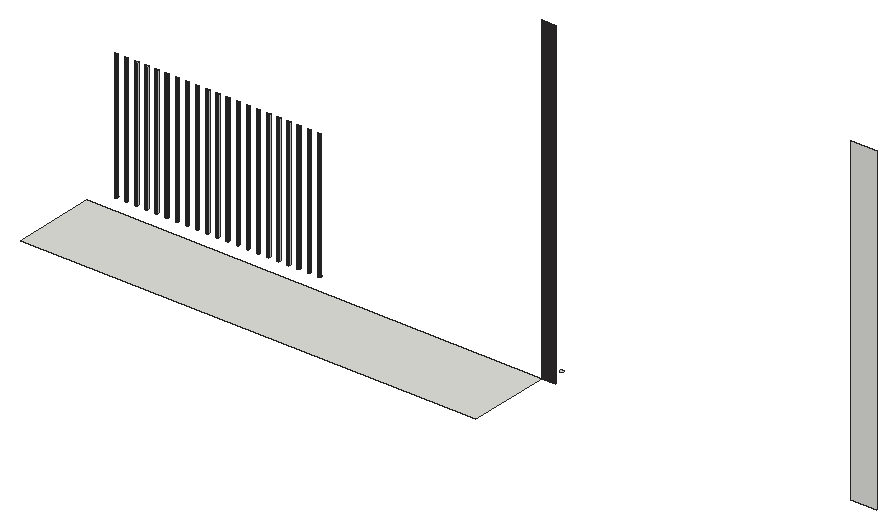
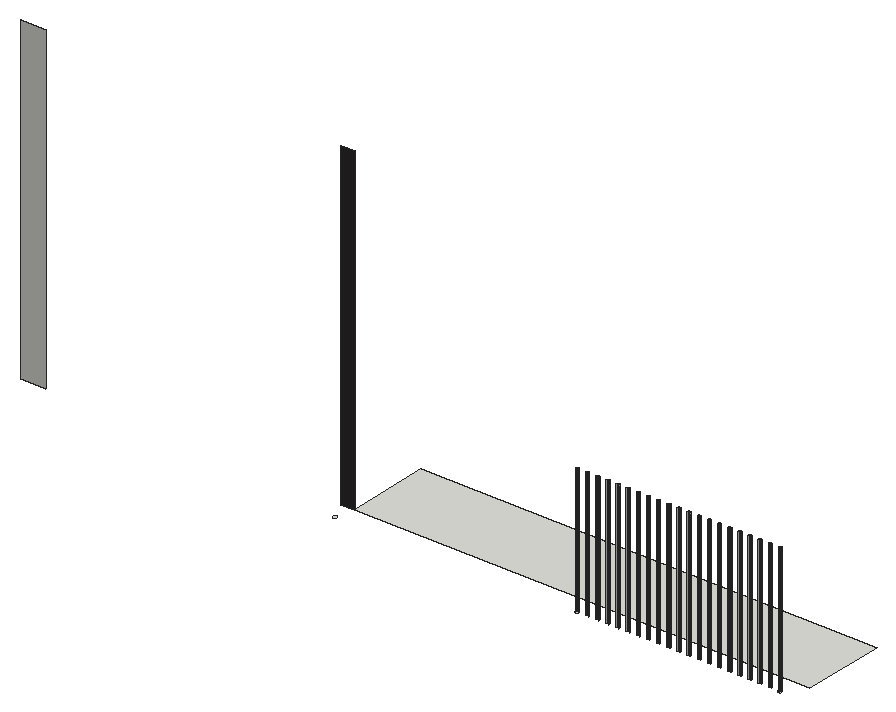
# SketchUp Ruby script. Lengths in inches.
U = 1.inch
M = Sketchup.active_model
def pt(a) = Geom::Point3d.new(a.map { |v| v * U })
def face(e, loops, mat)
  f = e.add_face(loops[0].map { |a| pt(a) })
  loops[1..].each { |l| e.add_face(l.map { |a| pt(a) }).erase! }
  f.material = f.back_material = mat if mat
  f
end
# faces: each face lists its corners as indices into pts; further lists are holes
def faces(e, pts, list, mat = nil) = list.each { |f| face(e, (f[0].is_a?(Array) ? f : [f]).map { |l| l.map { |i| pts[i] } }, mat) }
# xy, xz, yz: faces in a plane at the given z, y or x. An outline is a flat list of corners, or four numbers for a rectangle; further outlines are holes
def ring(l) = l.size == 4 ? [[l[0], l[1]], [l[2], l[1]], [l[2], l[3]], [l[0], l[3]]] : l.each_slice(2).to_a
def flat(e, list, mat, &to3) = list.each { |f| face(e, (f[0].is_a?(Array) ? f : [f]).map { |l| ring(l).map { |u, v| to3.(u, v) } }, mat) }
def xy(e, z, list, mat = nil) = flat(e, list, mat) { |x, y| [x, y, z] }
def xz(e, y, list, mat = nil) = flat(e, list, mat) { |x, z| [x, y, z] }
def yz(e, x, list, mat = nil) = flat(e, list, mat) { |y, z| [x, y, z] }
def lines(e, pts, list) = list.each { |a, b| e.add_line(pt(pts[a]), pt(pts[b])) }
# prism: a flat outline (further loops are holes) pulled along v
def prism(e, loops, v, mat = nil)
  f = face(e, loops, mat); d = Geom::Vector3d.new(v.map { |x| x * U })
  f.pushpull(f.normal.samedirection?(d) ? d.length : -d.length)
end
def box(e, o, s, mat = nil) = prism(e, [[o, [o[0] + s[0], o[1], o[2]], [o[0] + s[0], o[1] + s[1], o[2]], [o[0], o[1] + s[1], o[2]]]], [0, 0, s[2]], mat)
def at(x, y, z, deg = 0) = Geom::Transformation.translation(pt([x, y, z])) * Geom::Transformation.rotation(ORIGIN, Z_AXIS, deg.degrees)
def axes(o, x, y, z) = Geom::Transformation.new([*x, 0, *y, 0, *z, 0, *pt(o).to_a, 1])
def part(name) = M.definitions.add(name)
# library, detail: a bought-in or finely detailed component or shape, given as its bounding box
def library(name, o, s) = part(name).tap { |d| box(d.entities, o, s) }
def detail(e, o, s) = box(e.add_group.entities, o, s)
def put(e, d, t, mat = nil) = e.add_instance(d, t).tap { |i| i.material = mat if mat }
def group(e, t, mat = nil) = e.add_group.tap { |g| g.transformation = t; g.material = mat if mat }.entities
root = M.entities
M.materials.add("Generic\#4").color = [48, 45, 45]
xy(root,409.875,[[290.4375,81.125,528.75,124.5],[298.29,133.41,298.08,133.44,297.89,133.52,297.72,133.65,297.59,133.82,297.51,134.02,297.48,134.23,297.51,134.4375,297.59,134.63,297.72,134.8,297.89,134.93,298.08,135.01,298.29,135.04,298.5,135.01,298.7,134.93,298.87,134.8,299,134.63,299.08,134.4375,299.11,134.23,299.08,134.02,299,133.82,298.87,133.65,298.7,133.52,298.5,133.44],[404.54,133.41,404.33,133.44,404.14,133.52,403.97,133.65,403.84,133.82,403.76,134.02,403.73,134.23,403.76,134.4375,403.84,134.63,403.97,134.8,404.14,134.93,404.33,135.01,404.54,135.04,404.75,135.01,404.95,134.93,405.12,134.8,405.25,134.63,405.33,134.4375,405.36,134.23,405.33,134.02,405.25,133.82,405.12,133.65,404.95,133.52,404.75,133.44],[531.17,133.41,530.96,133.44,530.76,133.52,530.59,133.65,530.46,133.82,530.38,134.02,530.36,134.23,530.38,134.4375,530.46,134.63,530.59,134.8,530.76,134.93,530.96,135.01,531.17,135.04,531.38,135.01,531.57,134.93,531.74,134.8,531.87,134.63,531.95,134.4375,531.98,134.23,531.95,134.02,531.87,133.82,531.74,133.65,531.57,133.52,531.38,133.44]])
xz(root,124.5,[[690.4375,409.875,703.6875,577.875]])
xz(root,124.5,[[528.75,409.875,535.75,577.875]],"Generic\#4")
p = [[297.89,133.52,409.875],[298.08,133.44,409.875],[298.08,133.44,477.08],[297.89,133.52,477.08],[298.29,133.41,409.875],[298.29,133.41,477.08],
  [298.5,133.44,409.875],[298.5,133.44,477.08],[298.7,133.52,409.875],[298.7,133.52,477.08],[303.2,133.52,409.875],[303.4,133.44,409.875],
  [303.4,133.44,477.08],[303.2,133.52,477.08],[303.61,133.41,409.875],[303.61,133.41,477.08],[303.82,133.44,409.875],[303.82,133.44,477.08],
  [304.01,133.52,409.875],[304.01,133.52,477.08],[308.51,133.52,409.875],[308.71,133.44,409.875],[308.71,133.44,477.08],[308.51,133.52,477.08],
  [308.92,133.41,409.875],[308.92,133.41,477.08],[309.13,133.44,409.875],[309.13,133.44,477.08],[309.32,133.52,409.875],[309.32,133.52,477.08],
  [313.82,133.52,409.875],[314.02,133.44,409.875],[314.02,133.44,477.08],[313.82,133.52,477.08],[314.23,133.41,409.875],[314.23,133.41,477.08],
  [314.44,133.44,409.875],[314.44,133.44,477.08],[314.64,133.52,409.875],[314.64,133.52,477.08],[319.14,133.52,409.875],[319.33,133.44,409.875],
  [319.33,133.44,477.08],[319.14,133.52,477.08],[319.54,133.41,409.875],[319.54,133.41,477.08],[319.75,133.44,409.875],[319.75,133.44,477.08],
  [319.95,133.52,409.875],[319.95,133.52,477.08],[324.45,133.52,409.875],[324.65,133.44,409.875],[324.65,133.44,477.08],[324.45,133.52,477.08],
  [324.86,133.41,409.875],[324.86,133.41,477.08],[325.07,133.44,409.875],[325.07,133.44,477.08],[325.26,133.52,409.875],[325.26,133.52,477.08],
  [329.76,133.52,409.875],[329.96,133.44,409.875],[329.96,133.44,477.08],[329.76,133.52,477.08],[330.17,133.41,409.875],[330.17,133.41,477.08],
  [330.38,133.44,409.875],[330.38,133.44,477.08],[330.57,133.52,409.875],[330.57,133.52,477.08],[335.07,133.52,409.875],[335.27,133.44,409.875],
  [335.27,133.44,477.08],[335.07,133.52,477.08],[335.48,133.41,409.875],[335.48,133.41,477.08],[335.69,133.44,409.875],[335.69,133.44,477.08],
  [335.89,133.52,409.875],[335.89,133.52,477.08],[340.39,133.52,409.875],[340.58,133.44,409.875],[340.58,133.44,477.08],[340.39,133.52,477.08],
  [340.79,133.41,409.875],[340.79,133.41,477.08],[341,133.44,409.875],[341,133.44,477.08],[341.2,133.52,409.875],[341.2,133.52,477.08],
  [345.7,133.52,409.875],[345.9,133.44,409.875],[345.9,133.44,477.08],[345.7,133.52,477.08],[346.11,133.41,409.875],[346.11,133.41,477.08],
  [346.32,133.44,409.875],[346.32,133.44,477.08],[346.51,133.52,409.875],[346.51,133.52,477.08],[351.01,133.52,409.875],[351.21,133.44,409.875],
  [351.21,133.44,477.08],[351.01,133.52,477.08],[351.42,133.41,409.875],[351.42,133.41,477.08],[351.63,133.44,409.875],[351.63,133.44,477.08],
  [351.82,133.52,409.875],[351.82,133.52,477.08],[356.32,133.52,409.875],[356.52,133.44,409.875],[356.52,133.44,477.08],[356.32,133.52,477.08],
  [356.73,133.41,409.875],[356.73,133.41,477.08],[356.94,133.44,409.875],[356.94,133.44,477.08],[357.14,133.52,409.875],[357.14,133.52,477.08],
  [361.64,133.52,409.875],[361.83,133.44,409.875],[361.83,133.44,477.08],[361.64,133.52,477.08],[362.04,133.41,409.875],[362.04,133.41,477.08],
  [362.25,133.44,409.875],[362.25,133.44,477.08],[362.45,133.52,409.875],[362.45,133.52,477.08],[366.95,133.52,409.875],[367.15,133.44,409.875],
  [367.15,133.44,477.08],[366.95,133.52,477.08],[367.36,133.41,409.875],[367.36,133.41,477.08],[367.57,133.44,409.875],[367.57,133.44,477.08],
  [367.76,133.52,409.875],[367.76,133.52,477.08],[372.26,133.52,409.875],[372.46,133.44,409.875],[372.46,133.44,477.08],[372.26,133.52,477.08],
  [372.67,133.41,409.875],[372.67,133.41,477.08],[372.88,133.44,409.875],[372.88,133.44,477.08],[373.07,133.52,409.875],[373.07,133.52,477.08],
  [377.57,133.52,409.875],[377.77,133.44,409.875],[377.77,133.44,477.08],[377.57,133.52,477.08],[377.98,133.41,409.875],[377.98,133.41,477.08],
  [378.19,133.44,409.875],[378.19,133.44,477.08],[378.39,133.52,409.875],[378.39,133.52,477.08],[382.89,133.52,409.875],[383.08,133.44,409.875],
  [383.08,133.44,477.08],[382.89,133.52,477.08],[383.29,133.41,409.875],[383.29,133.41,477.08],[383.5,133.44,409.875],[383.5,133.44,477.08],
  [383.7,133.52,409.875],[383.7,133.52,477.08],[388.2,133.52,409.875],[388.4,133.44,409.875],[388.4,133.44,477.08],[388.2,133.52,477.08],
  [388.61,133.41,409.875],[388.61,133.41,477.08],[388.82,133.44,409.875],[388.82,133.44,477.08],[389.01,133.52,409.875],[389.01,133.52,477.08],
  [393.51,133.52,409.875],[393.71,133.44,409.875],[393.71,133.44,477.08],[393.51,133.52,477.08],[393.92,133.41,409.875],[393.92,133.41,477.08],
  [394.13,133.44,409.875],[394.13,133.44,477.08],[394.32,133.52,409.875],[394.32,133.52,477.08],[398.82,133.52,409.875],[399.02,133.44,409.875],
  [399.02,133.44,477.08],[398.82,133.52,477.08],[399.23,133.41,409.875],[399.23,133.41,477.08],[399.44,133.44,409.875],[399.44,133.44,477.08],
  [399.64,133.52,409.875],[399.64,133.52,477.08],[404.14,133.52,409.875],[404.33,133.44,409.875],[404.33,133.44,477.08],[404.14,133.52,477.08],
  [404.54,133.41,409.875],[404.54,133.41,477.08],[404.75,133.44,409.875],[404.75,133.44,477.08],[404.95,133.52,409.875],[404.95,133.52,477.08],
  [297.72,133.65,409.875],[297.72,133.65,477.08],[298.87,133.65,409.875],[298.87,133.65,477.08],[303.03,133.65,409.875],[303.03,133.65,477.08],
  [304.18,133.65,409.875],[304.18,133.65,477.08],[308.34,133.65,409.875],[308.34,133.65,477.08],[309.49,133.65,409.875],[309.49,133.65,477.08],
  [313.66,133.65,409.875],[313.66,133.65,477.08],[314.8,133.65,409.875],[314.8,133.65,477.08],[318.97,133.65,409.875],[318.97,133.65,477.08],
  [320.12,133.65,409.875],[320.12,133.65,477.08],[324.28,133.65,409.875],[324.28,133.65,477.08],[325.43,133.65,409.875],[325.43,133.65,477.08],
  [329.59,133.65,409.875],[329.59,133.65,477.08],[330.74,133.65,409.875],[330.74,133.65,477.08],[334.91,133.65,409.875],[334.91,133.65,477.08],
  [336.05,133.65,409.875],[336.05,133.65,477.08],[340.22,133.65,409.875],[340.22,133.65,477.08],[341.37,133.65,409.875],[341.37,133.65,477.08],
  [345.53,133.65,409.875],[345.53,133.65,477.08],[346.68,133.65,409.875],[346.68,133.65,477.08],[350.84,133.65,409.875],[350.84,133.65,477.08],
  [351.99,133.65,409.875],[351.99,133.65,477.08],[356.16,133.65,409.875],[356.16,133.65,477.08],[357.3,133.65,409.875],[357.3,133.65,477.08],
  [361.47,133.65,409.875],[361.47,133.65,477.08],[362.62,133.65,409.875],[362.62,133.65,477.08],[366.78,133.65,409.875],[366.78,133.65,477.08],
  [367.93,133.65,409.875],[367.93,133.65,477.08],[372.09,133.65,409.875],[372.09,133.65,477.08],[373.24,133.65,409.875],[373.24,133.65,477.08],
  [377.41,133.65,409.875],[377.41,133.65,477.08],[378.55,133.65,409.875],[378.55,133.65,477.08],[382.72,133.65,409.875],[382.72,133.65,477.08],
  [383.87,133.65,409.875],[383.87,133.65,477.08],[388.03,133.65,409.875],[388.03,133.65,477.08],[389.18,133.65,409.875],[389.18,133.65,477.08],
  [393.34,133.65,409.875],[393.34,133.65,477.08],[394.49,133.65,409.875],[394.49,133.65,477.08],[398.66,133.65,409.875],[398.66,133.65,477.08],
  [399.8,133.65,409.875],[399.8,133.65,477.08],[403.97,133.65,409.875],[403.97,133.65,477.08],[405.12,133.65,409.875],[405.12,133.65,477.08],
  [297.59,133.82,409.875],[297.59,133.82,477.08],[299,133.82,409.875],[299,133.82,477.08],[302.9,133.82,409.875],[302.9,133.82,477.08],
  [304.31,133.82,409.875],[304.31,133.82,477.08],[308.21,133.82,409.875],[308.21,133.82,477.08],[309.62,133.82,409.875],[309.62,133.82,477.08],
  [313.53,133.82,409.875],[313.53,133.82,477.08],[314.93,133.82,409.875],[314.93,133.82,477.08],[318.84,133.82,409.875],[318.84,133.82,477.08],
  [320.25,133.82,409.875],[320.25,133.82,477.08],[324.15,133.82,409.875],[324.15,133.82,477.08],[325.56,133.82,409.875],[325.56,133.82,477.08],
  [329.46,133.82,409.875],[329.46,133.82,477.08],[330.87,133.82,409.875],[330.87,133.82,477.08],[334.78,133.82,409.875],[334.78,133.82,477.08],
  [336.18,133.82,409.875],[336.18,133.82,477.08],[340.09,133.82,409.875],[340.09,133.82,477.08],[341.5,133.82,409.875],[341.5,133.82,477.08],
  [345.4,133.82,409.875],[345.4,133.82,477.08],[346.81,133.82,409.875],[346.81,133.82,477.08],[350.71,133.82,409.875],[350.71,133.82,477.08],
  [352.12,133.82,409.875],[352.12,133.82,477.08],[356.03,133.82,409.875],[356.03,133.82,477.08],[357.43,133.82,409.875],[357.43,133.82,477.08],
  [361.34,133.82,409.875],[361.34,133.82,477.08],[362.75,133.82,409.875],[362.75,133.82,477.08],[366.65,133.82,409.875],[366.65,133.82,477.08],
  [368.06,133.82,409.875],[368.06,133.82,477.08],[371.96,133.82,409.875],[371.96,133.82,477.08],[373.37,133.82,409.875],[373.37,133.82,477.08],
  [377.28,133.82,409.875],[377.28,133.82,477.08],[378.68,133.82,409.875],[378.68,133.82,477.08],[382.59,133.82,409.875],[382.59,133.82,477.08],
  [384,133.82,409.875],[384,133.82,477.08],[387.9,133.82,409.875],[387.9,133.82,477.08],[389.31,133.82,409.875],[389.31,133.82,477.08],
  [393.21,133.82,409.875],[393.21,133.82,477.08],[394.62,133.82,409.875],[394.62,133.82,477.08],[398.53,133.82,409.875],[398.53,133.82,477.08],
  [399.93,133.82,409.875],[399.93,133.82,477.08],[403.84,133.82,409.875],[403.84,133.82,477.08],[405.25,133.82,409.875],[405.25,133.82,477.08],
  [297.51,134.02,409.875],[297.51,134.02,477.08],[299.08,134.02,409.875],[299.08,134.02,477.08],[302.82,134.02,409.875],[302.82,134.02,477.08],
  [304.39,134.02,409.875],[304.39,134.02,477.08],[308.13,134.02,409.875],[308.13,134.02,477.08],[309.7,134.02,409.875],[309.7,134.02,477.08],
  [313.45,134.02,409.875],[313.45,134.02,477.08],[315.02,134.02,409.875],[315.02,134.02,477.08],[318.76,134.02,409.875],[318.76,134.02,477.08],
  [320.33,134.02,409.875],[320.33,134.02,477.08],[324.07,134.02,409.875],[324.07,134.02,477.08],[325.64,134.02,409.875],[325.64,134.02,477.08],
  [329.38,134.02,409.875],[329.38,134.02,477.08],[330.95,134.02,409.875],[330.95,134.02,477.08],[334.7,134.02,409.875],[334.7,134.02,477.08],
  [336.27,134.02,409.875],[336.27,134.02,477.08],[340.01,134.02,409.875],[340.01,134.02,477.08],[341.58,134.02,409.875],[341.58,134.02,477.08],
  [345.32,134.02,409.875],[345.32,134.02,477.08],[346.89,134.02,409.875],[346.89,134.02,477.08],[350.63,134.02,409.875],[350.63,134.02,477.08],
  [352.2,134.02,409.875],[352.2,134.02,477.08],[355.95,134.02,409.875],[355.95,134.02,477.08],[357.52,134.02,409.875],[357.52,134.02,477.08],
  [361.26,134.02,409.875],[361.26,134.02,477.08],[362.83,134.02,409.875],[362.83,134.02,477.08],[366.57,134.02,409.875],[366.57,134.02,477.08],
  [368.14,134.02,409.875],[368.14,134.02,477.08],[371.88,134.02,409.875],[371.88,134.02,477.08],[373.45,134.02,409.875],[373.45,134.02,477.08],
  [377.2,134.02,409.875],[377.2,134.02,477.08],[378.77,134.02,409.875],[378.77,134.02,477.08],[382.51,134.02,409.875],[382.51,134.02,477.08],
  [384.08,134.02,409.875],[384.08,134.02,477.08],[387.82,134.02,409.875],[387.82,134.02,477.08],[389.39,134.02,409.875],[389.39,134.02,477.08],
  [393.13,134.02,409.875],[393.13,134.02,477.08],[394.7,134.02,409.875],[394.7,134.02,477.08],[398.45,134.02,409.875],[398.45,134.02,477.08],
  [400.02,134.02,409.875],[400.02,134.02,477.08],[403.76,134.02,409.875],[403.76,134.02,477.08],[405.33,134.02,409.875],[405.33,134.02,477.08],
  [297.48,134.23,409.875],[297.48,134.23,477.08],[299.11,134.23,409.875],[299.11,134.23,477.08],[302.79,134.23,409.875],[302.79,134.23,477.08],
  [304.42,134.23,409.875],[304.42,134.23,477.08],[308.11,134.23,409.875],[308.11,134.23,477.08],[309.73,134.23,409.875],[309.73,134.23,477.08],
  [313.42,134.23,409.875],[313.42,134.23,477.08],[315.04,134.23,409.875],[315.04,134.23,477.08],[318.73,134.23,409.875],[318.73,134.23,477.08],
  [320.36,134.23,409.875],[320.36,134.23,477.08],[324.04,134.23,409.875],[324.04,134.23,477.08],[325.67,134.23,409.875],[325.67,134.23,477.08],
  [329.36,134.23,409.875],[329.36,134.23,477.08],[330.98,134.23,409.875],[330.98,134.23,477.08],[334.67,134.23,409.875],[334.67,134.23,477.08],
  [336.29,134.23,409.875],[336.29,134.23,477.08],[339.98,134.23,409.875],[339.98,134.23,477.08],[341.61,134.23,409.875],[341.61,134.23,477.08],
  [345.29,134.23,409.875],[345.29,134.23,477.08],[346.92,134.23,409.875],[346.92,134.23,477.08],[350.61,134.23,409.875],[350.61,134.23,477.08],
  [352.23,134.23,409.875],[352.23,134.23,477.08],[355.92,134.23,409.875],[355.92,134.23,477.08],[357.54,134.23,409.875],[357.54,134.23,477.08],
  [361.23,134.23,409.875],[361.23,134.23,477.08],[362.86,134.23,409.875],[362.86,134.23,477.08],[366.54,134.23,409.875],[366.54,134.23,477.08],
  [368.17,134.23,409.875],[368.17,134.23,477.08],[371.86,134.23,409.875],[371.86,134.23,477.08],[373.48,134.23,409.875],[373.48,134.23,477.08],
  [377.17,134.23,409.875],[377.17,134.23,477.08],[378.79,134.23,409.875],[378.79,134.23,477.08],[382.48,134.23,409.875],[382.48,134.23,477.08],
  [384.11,134.23,409.875],[384.11,134.23,477.08],[387.79,134.23,409.875],[387.79,134.23,477.08],[389.42,134.23,409.875],[389.42,134.23,477.08],
  [393.11,134.23,409.875],[393.11,134.23,477.08],[394.73,134.23,409.875],[394.73,134.23,477.08],[398.42,134.23,409.875],[398.42,134.23,477.08],
  [400.04,134.23,409.875],[400.04,134.23,477.08],[403.73,134.23,409.875],[403.73,134.23,477.08],[405.36,134.23,409.875],[405.36,134.23,477.08]]
faces(root,p,[[0,1,2,3],[1,4,5,2],[4,6,7,5],[6,8,9,7],[10,11,12,13],[11,14,15,12],[14,16,17,15],[16,18,19,17],
  [20,21,22,23],[21,24,25,22],[24,26,27,25],[26,28,29,27],[30,31,32,33],[31,34,35,32],[34,36,37,35],[36,38,39,37],
  [40,41,42,43],[41,44,45,42],[44,46,47,45],[46,48,49,47],[50,51,52,53],[51,54,55,52],[54,56,57,55],[56,58,59,57],
  [60,61,62,63],[61,64,65,62],[64,66,67,65],[66,68,69,67],[70,71,72,73],[71,74,75,72],[74,76,77,75],[76,78,79,77],
  [80,81,82,83],[81,84,85,82],[84,86,87,85],[86,88,89,87],[90,91,92,93],[91,94,95,92],[94,96,97,95],[96,98,99,97],
  [100,101,102,103],[101,104,105,102],[104,106,107,105],[106,108,109,107],[110,111,112,113],[111,114,115,112],[114,116,117,115],[116,118,119,117],
  [120,121,122,123],[121,124,125,122],[124,126,127,125],[126,128,129,127],[130,131,132,133],[131,134,135,132],[134,136,137,135],[136,138,139,137],
  [140,141,142,143],[141,144,145,142],[144,146,147,145],[146,148,149,147],[150,151,152,153],[151,154,155,152],[154,156,157,155],[156,158,159,157],
  [160,161,162,163],[161,164,165,162],[164,166,167,165],[166,168,169,167],[170,171,172,173],[171,174,175,172],[174,176,177,175],[176,178,179,177],
  [180,181,182,183],[181,184,185,182],[184,186,187,185],[186,188,189,187],[190,191,192,193],[191,194,195,192],[194,196,197,195],[196,198,199,197],
  [200,201,202,203],[201,204,205,202],[204,206,207,205],[206,208,209,207],[210,0,3,211],[8,212,213,9],[214,10,13,215],[18,216,217,19],
  [218,20,23,219],[28,220,221,29],[222,30,33,223],[38,224,225,39],[226,40,43,227],[48,228,229,49],[230,50,53,231],[58,232,233,59],
  [234,60,63,235],[68,236,237,69],[238,70,73,239],[78,240,241,79],[242,80,83,243],[88,244,245,89],[246,90,93,247],[98,248,249,99],
  [250,100,103,251],[108,252,253,109],[254,110,113,255],[118,256,257,119],[258,120,123,259],[128,260,261,129],[262,130,133,263],[138,264,265,139],
  [266,140,143,267],[148,268,269,149],[270,150,153,271],[158,272,273,159],[274,160,163,275],[168,276,277,169],[278,170,173,279],[178,280,281,179],
  [282,180,183,283],[188,284,285,189],[286,190,193,287],[198,288,289,199],[290,200,203,291],[208,292,293,209],[294,210,211,295],[212,296,297,213],
  [298,214,215,299],[216,300,301,217],[302,218,219,303],[220,304,305,221],[306,222,223,307],[224,308,309,225],[310,226,227,311],[228,312,313,229],
  [314,230,231,315],[232,316,317,233],[318,234,235,319],[236,320,321,237],[322,238,239,323],[240,324,325,241],[326,242,243,327],[244,328,329,245],
  [330,246,247,331],[248,332,333,249],[334,250,251,335],[252,336,337,253],[338,254,255,339],[256,340,341,257],[342,258,259,343],[260,344,345,261],
  [346,262,263,347],[264,348,349,265],[350,266,267,351],[268,352,353,269],[354,270,271,355],[272,356,357,273],[358,274,275,359],[276,360,361,277],
  [362,278,279,363],[280,364,365,281],[366,282,283,367],[284,368,369,285],[370,286,287,371],[288,372,373,289],[374,290,291,375],[292,376,377,293],
  [378,294,295,379],[296,380,381,297],[382,298,299,383],[300,384,385,301],[386,302,303,387],[304,388,389,305],[390,306,307,391],[308,392,393,309],
  [394,310,311,395],[312,396,397,313],[398,314,315,399],[316,400,401,317],[402,318,319,403],[320,404,405,321],[406,322,323,407],[324,408,409,325],
  [410,326,327,411],[328,412,413,329],[414,330,331,415],[332,416,417,333],[418,334,335,419],[336,420,421,337],[422,338,339,423],[340,424,425,341],
  [426,342,343,427],[344,428,429,345],[430,346,347,431],[348,432,433,349],[434,350,351,435],[352,436,437,353],[438,354,355,439],[356,440,441,357],
  [442,358,359,443],[360,444,445,361],[446,362,363,447],[364,448,449,365],[450,366,367,451],[368,452,453,369],[454,370,371,455],[372,456,457,373],
  [458,374,375,459],[376,460,461,377],[462,378,379,463],[380,464,465,381],[466,382,383,467],[384,468,469,385],[470,386,387,471],[388,472,473,389],
  [474,390,391,475],[392,476,477,393],[478,394,395,479],[396,480,481,397],[482,398,399,483],[400,484,485,401],[486,402,403,487],[404,488,489,405],
  [490,406,407,491],[408,492,493,409],[494,410,411,495],[412,496,497,413],[498,414,415,499],[416,500,501,417],[502,418,419,503],[420,504,505,421],
  [506,422,423,507],[424,508,509,425],[510,426,427,511],[428,512,513,429],[514,430,431,515],[432,516,517,433],[518,434,435,519],[436,520,521,437],
  [522,438,439,523],[440,524,525,441],[526,442,443,527],[444,528,529,445],[530,446,447,531],[448,532,533,449],[534,450,451,535],[452,536,537,453],
  [538,454,455,539],[456,540,541,457],[542,458,459,543],[460,544,545,461]])
